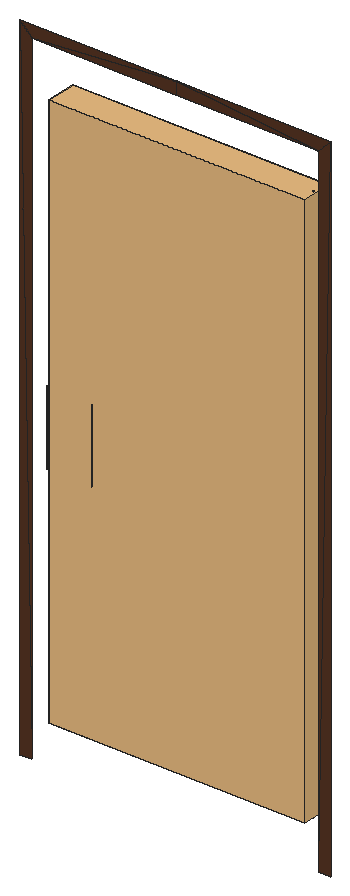
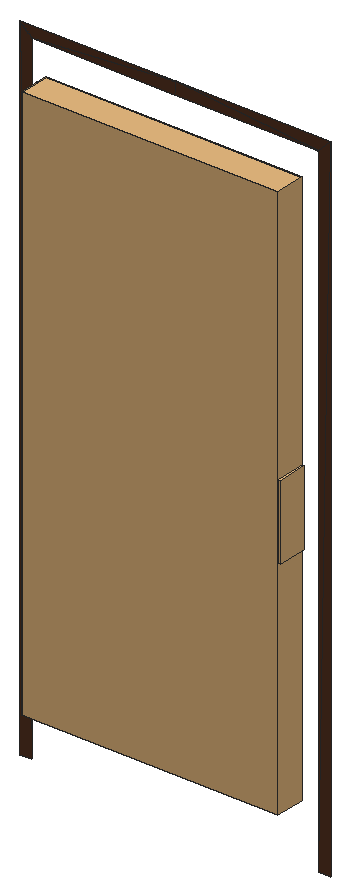
# SketchUp Ruby script. Lengths in inches.
U = 1.inch
M = Sketchup.active_model
def pt(a) = Geom::Point3d.new(a.map { |v| v * U })
def face(e, loops, mat)
  f = e.add_face(loops[0].map { |a| pt(a) })
  loops[1..].each { |l| e.add_face(l.map { |a| pt(a) }).erase! }
  f.material = f.back_material = mat if mat
  f
end
# faces: each face lists its corners as indices into pts; further lists are holes
def faces(e, pts, list, mat = nil) = list.each { |f| face(e, (f[0].is_a?(Array) ? f : [f]).map { |l| l.map { |i| pts[i] } }, mat) }
# xy, xz, yz: faces in a plane at the given z, y or x. An outline is a flat list of corners, or four numbers for a rectangle; further outlines are holes
def ring(l) = l.size == 4 ? [[l[0], l[1]], [l[2], l[1]], [l[2], l[3]], [l[0], l[3]]] : l.each_slice(2).to_a
def flat(e, list, mat, &to3) = list.each { |f| face(e, (f[0].is_a?(Array) ? f : [f]).map { |l| ring(l).map { |u, v| to3.(u, v) } }, mat) }
def xy(e, z, list, mat = nil) = flat(e, list, mat) { |x, y| [x, y, z] }
def xz(e, y, list, mat = nil) = flat(e, list, mat) { |x, z| [x, y, z] }
def yz(e, x, list, mat = nil) = flat(e, list, mat) { |y, z| [x, y, z] }
def lines(e, pts, list) = list.each { |a, b| e.add_line(pt(pts[a]), pt(pts[b])) }
# prism: a flat outline (further loops are holes) pulled along v
def prism(e, loops, v, mat = nil)
  f = face(e, loops, mat); d = Geom::Vector3d.new(v.map { |x| x * U })
  f.pushpull(f.normal.samedirection?(d) ? d.length : -d.length)
end
def box(e, o, s, mat = nil) = prism(e, [[o, [o[0] + s[0], o[1], o[2]], [o[0] + s[0], o[1] + s[1], o[2]], [o[0], o[1] + s[1], o[2]]]], [0, 0, s[2]], mat)
def at(x, y, z, deg = 0) = Geom::Transformation.translation(pt([x, y, z])) * Geom::Transformation.rotation(ORIGIN, Z_AXIS, deg.degrees)
def axes(o, x, y, z) = Geom::Transformation.new([*x, 0, *y, 0, *z, 0, *pt(o).to_a, 1])
def part(name) = M.definitions.add(name)
# library, detail: a bought-in or finely detailed component or shape, given as its bounding box
def library(name, o, s) = part(name).tap { |d| box(d.entities, o, s) }
def detail(e, o, s) = box(e.add_group.entities, o, s)
def put(e, d, t, mat = nil) = e.add_instance(d, t).tap { |i| i.material = mat if mat }
def group(e, t, mat = nil) = e.add_group.tap { |g| g.transformation = t; g.material = mat if mat }.entities
root = M.entities
M.materials.add("Material \#0").color = [86, 53, 35]
M.materials.add("Material \#1").color = [140, 140, 140]
c1 = part("3DGeom~8_Defintion")
xz(c1.entities,-471.94,[[458.125,-17.29,459.53,-16.11,457.73,-17.15],[458.125,-17.29,458.54,-17.29,459.53,-16.11],[458.54,-17.29,458.93,-17.15,459.53,-16.11],[457.73,-17.15,459.53,-16.11,457.42,-16.88],[458.93,-17.15,459.25,-16.88,459.53,-16.11],
  [457.42,-16.88,459.53,-16.11,457.21,-16.52],[459.25,-16.88,459.46,-16.52,459.53,-16.11],[457.21,-16.52,459.53,-16.11,457.14,-16.11],[457.14,-16.11,459.53,-16.11,457.21,-15.7],[459.53,-16.11,457.42,-15.34,457.21,-15.7],
  [459.53,-16.11,457.73,-15.07,457.42,-15.34],[459.53,-16.11,458.125,-14.93,457.73,-15.07],[459.53,-16.11,458.54,-14.93,458.125,-14.93],[459.53,-16.11,458.93,-15.07,458.54,-14.93],[459.53,-16.11,459.25,-15.34,458.93,-15.07],
  [459.53,-16.11,459.46,-15.7,459.25,-15.34]],"Material \#1")
xz(c1.entities,-416.39,[[458.125,-17.29,457.73,-17.15,459.53,-16.11],[458.125,-17.29,459.53,-16.11,458.54,-17.29],[458.54,-17.29,459.53,-16.11,458.93,-17.15],[457.73,-17.15,457.42,-16.88,459.53,-16.11],[458.93,-17.15,459.53,-16.11,459.25,-16.88],
  [457.42,-16.88,457.21,-16.52,459.53,-16.11],[459.25,-16.88,459.53,-16.11,459.46,-16.52],[457.21,-16.52,457.14,-16.11,459.53,-16.11],[457.14,-16.11,457.21,-15.7,459.53,-16.11],[459.53,-16.11,457.21,-15.7,457.42,-15.34],
  [459.53,-16.11,457.42,-15.34,457.73,-15.07],[459.53,-16.11,457.73,-15.07,458.125,-14.93],[459.53,-16.11,458.125,-14.93,458.54,-14.93],[459.53,-16.11,458.54,-14.93,458.93,-15.07],[459.53,-16.11,458.93,-15.07,459.25,-15.34],
  [459.53,-16.11,459.25,-15.34,459.46,-15.7]],"Material \#1")
xz(c1.entities,-27.5,[[458.125,-17.29,459.53,-16.11,457.73,-17.15],[458.125,-17.29,458.54,-17.29,459.53,-16.11],[458.54,-17.29,458.93,-17.15,459.53,-16.11],[457.73,-17.15,459.53,-16.11,457.42,-16.88],[458.93,-17.15,459.25,-16.88,459.53,-16.11],
  [457.42,-16.88,459.53,-16.11,457.21,-16.52],[459.25,-16.88,459.46,-16.52,459.53,-16.11],[457.21,-16.52,459.53,-16.11,457.14,-16.11],[457.14,-16.11,459.53,-16.11,457.21,-15.7],[459.53,-16.11,457.42,-15.34,457.21,-15.7],
  [459.53,-16.11,457.73,-15.07,457.42,-15.34],[459.53,-16.11,458.125,-14.93,457.73,-15.07],[459.53,-16.11,458.54,-14.93,458.125,-14.93],[459.53,-16.11,458.93,-15.07,458.54,-14.93],[459.53,-16.11,459.25,-15.34,458.93,-15.07],
  [459.53,-16.11,459.46,-15.7,459.25,-15.34]],"Material \#1")
xz(c1.entities,28.06,[[458.125,-17.29,457.73,-17.15,459.53,-16.11],[458.125,-17.29,459.53,-16.11,458.54,-17.29],[458.54,-17.29,459.53,-16.11,458.93,-17.15],[457.73,-17.15,457.42,-16.88,459.53,-16.11],[458.93,-17.15,459.53,-16.11,459.25,-16.88],
  [457.42,-16.88,457.21,-16.52,459.53,-16.11],[459.25,-16.88,459.53,-16.11,459.46,-16.52],[457.21,-16.52,457.14,-16.11,459.53,-16.11],[457.14,-16.11,457.21,-15.7,459.53,-16.11],[459.53,-16.11,457.21,-15.7,457.42,-15.34],
  [459.53,-16.11,457.42,-15.34,457.73,-15.07],[459.53,-16.11,457.73,-15.07,458.125,-14.93],[459.53,-16.11,458.125,-14.93,458.54,-14.93],[459.53,-16.11,458.54,-14.93,458.93,-15.07],[459.53,-16.11,458.93,-15.07,459.25,-15.34],
  [459.53,-16.11,459.25,-15.34,459.46,-15.7]],"Material \#1")
xz(c1.entities,472.5,[[458.125,-17.29,459.53,-16.11,457.73,-17.15],[458.125,-17.29,458.54,-17.29,459.53,-16.11],[458.54,-17.29,458.93,-17.15,459.53,-16.11],[457.73,-17.15,459.53,-16.11,457.42,-16.88],[458.93,-17.15,459.25,-16.88,459.53,-16.11],
  [457.42,-16.88,459.53,-16.11,457.21,-16.52],[459.25,-16.88,459.46,-16.52,459.53,-16.11],[457.21,-16.52,459.53,-16.11,457.14,-16.11],[457.14,-16.11,459.53,-16.11,457.21,-15.7],[459.53,-16.11,457.42,-15.34,457.21,-15.7],
  [459.53,-16.11,457.73,-15.07,457.42,-15.34],[459.53,-16.11,458.125,-14.93,457.73,-15.07],[459.53,-16.11,458.54,-14.93,458.125,-14.93],[459.53,-16.11,458.93,-15.07,458.54,-14.93],[459.53,-16.11,459.25,-15.34,458.93,-15.07],
  [459.53,-16.11,459.46,-15.7,459.25,-15.34]],"Material \#1")
xz(c1.entities,528.06,[[458.125,-17.29,457.73,-17.15,459.53,-16.11],[458.125,-17.29,459.53,-16.11,458.54,-17.29],[458.54,-17.29,459.53,-16.11,458.93,-17.15],[457.73,-17.15,457.42,-16.88,459.53,-16.11],[458.93,-17.15,459.53,-16.11,459.25,-16.88],
  [457.42,-16.88,457.21,-16.52,459.53,-16.11],[459.25,-16.88,459.53,-16.11,459.46,-16.52],[457.21,-16.52,457.14,-16.11,459.53,-16.11],[457.14,-16.11,457.21,-15.7,459.53,-16.11],[459.53,-16.11,457.21,-15.7,457.42,-15.34],
  [459.53,-16.11,457.42,-15.34,457.73,-15.07],[459.53,-16.11,457.73,-15.07,458.125,-14.93],[459.53,-16.11,458.125,-14.93,458.54,-14.93],[459.53,-16.11,458.54,-14.93,458.93,-15.07],[459.53,-16.11,458.93,-15.07,459.25,-15.34],
  [459.53,-16.11,459.25,-15.34,459.46,-15.7]],"Material \#1")
c2 = part("3DGeom~21_Defintion")
xy(c2.entities,73.08,[[-976.3,-241.71,23.7,-241.71,-976.3,-223.46],[23.7,-241.71,5.45,-223.46,-976.3,-223.46],[23.7,-241.71,23.7,0,5.45,-223.46],[5.45,-223.46,23.7,0,5.45,0],[23.7,0,23.7,241.71,5.45,223.46],
  [5.45,0,23.7,0,5.45,223.46],[-976.3,223.46,23.7,241.71,-976.3,241.71],[-976.3,223.46,5.45,223.46,23.7,241.71]],"Material \#0")
c3 = library("3DGeom~6_Defintion",[-5.59,-471.8,-48.03],[468.87,1000,73.72])
c4 = library("3DGeom~3_Defintion",[-83.33,-500,-350],[620.1,1000,533.33])
c5 = library("3DGeom~1_Defintion",[-60.87,347.29,-704.08],[121.74,121.75,1000])
c6 = library("3DGeom~13_Defintion",[-84.91,-744.98,-830.03],[169.82,169.83,1000])
xy(root,6.597,[[381.979,199.777,381.911,199.796,381.922,199.809],[381.979,199.777,381.922,199.809,381.983,199.793],[381.979,199.777,381.983,199.793,382.051,199.777],[382.051,199.777,381.983,199.793,382.047,199.793],[382.051,199.777,382.047,199.793,382.119,199.796],
  [382.047,199.793,382.108,199.809,382.119,199.796],[381.911,199.796,381.856,199.83,381.872,199.84],[381.911,199.796,381.872,199.84,381.922,199.809],[382.119,199.796,382.108,199.809,382.174,199.83],[382.108,199.809,382.158,199.84,382.174,199.83],
  [381.856,199.83,381.82,199.877,381.84,199.883],[381.856,199.83,381.84,199.883,381.872,199.84],[382.174,199.83,382.158,199.84,382.21,199.877],[382.158,199.84,382.19,199.883,382.21,199.877],[381.82,199.877,381.808,199.93,381.828,199.93],
  [381.82,199.877,381.828,199.93,381.84,199.883],[382.21,199.877,382.19,199.883,382.222,199.93],[382.19,199.883,382.201,199.93,382.222,199.93],[381.808,199.93,381.82,199.984,381.84,199.978],[381.808,199.93,381.84,199.978,381.828,199.93],
  [382.201,199.93,382.19,199.978,382.21,199.984],[382.201,199.93,382.21,199.984,382.222,199.93],[381.84,199.978,381.82,199.984,381.872,200.02],[382.19,199.978,382.158,200.02,382.174,200.03],[382.19,199.978,382.174,200.03,382.21,199.984],
  [381.82,199.984,381.856,200.03,381.872,200.02],[381.872,200.02,381.856,200.03,381.922,200.052],[382.158,200.02,382.108,200.052,382.119,200.065],[382.158,200.02,382.119,200.065,382.174,200.03],[381.856,200.03,381.911,200.065,381.922,200.052],
  [381.922,200.052,381.911,200.065,381.983,200.068],[382.108,200.052,382.047,200.068,382.051,200.084],[382.108,200.052,382.051,200.084,382.119,200.065],[381.911,200.065,381.979,200.084,381.983,200.068],[381.983,200.068,381.979,200.084,382.047,200.068],
  [382.047,200.068,381.979,200.084,382.051,200.084]],"Material \#1")
xy(root,6.614,[[381.979,199.777,381.983,199.793,381.911,199.796],[381.979,199.777,382.047,199.793,381.983,199.793],[381.979,199.777,382.051,199.777,382.047,199.793],[382.051,199.777,382.108,199.809,382.047,199.793],[382.051,199.777,382.119,199.796,382.108,199.809],
  [381.983,199.793,381.922,199.809,381.911,199.796],[381.911,199.796,381.922,199.809,381.856,199.83],[382.119,199.796,382.158,199.84,382.108,199.809],[382.119,199.796,382.174,199.83,382.158,199.84],[381.922,199.809,381.872,199.84,381.856,199.83],
  [381.856,199.83,381.872,199.84,381.82,199.877],[382.174,199.83,382.19,199.883,382.158,199.84],[382.174,199.83,382.21,199.877,382.19,199.883],[381.872,199.84,381.84,199.883,381.82,199.877],[381.82,199.877,381.84,199.883,381.808,199.93],
  [382.21,199.877,382.201,199.93,382.19,199.883],[382.21,199.877,382.222,199.93,382.201,199.93],[381.84,199.883,381.828,199.93,381.808,199.93],[381.808,199.93,381.828,199.93,381.82,199.984],[381.828,199.93,381.84,199.978,381.82,199.984],
  [382.201,199.93,382.222,199.93,382.19,199.978],[382.222,199.93,382.21,199.984,382.19,199.978],[381.84,199.978,381.856,200.03,381.82,199.984],[381.84,199.978,381.872,200.02,381.856,200.03],[382.19,199.978,382.21,199.984,382.158,200.02],
  [382.21,199.984,382.174,200.03,382.158,200.02],[381.872,200.02,381.911,200.065,381.856,200.03],[381.872,200.02,381.922,200.052,381.911,200.065],[382.158,200.02,382.174,200.03,382.108,200.052],[382.174,200.03,382.119,200.065,382.108,200.052],
  [381.922,200.052,381.979,200.084,381.911,200.065],[381.922,200.052,381.983,200.068,381.979,200.084],[382.108,200.052,382.119,200.065,382.047,200.068],[382.119,200.065,382.051,200.084,382.047,200.068],[381.983,200.068,382.051,200.084,381.979,200.084],
  [381.983,200.068,382.047,200.068,382.051,200.084]],"Material \#1")
xy(root,10.426,[[381.979,199.777,381.911,199.796,381.983,199.793],[381.979,199.777,381.983,199.793,382.047,199.793],[381.979,199.777,382.047,199.793,382.051,199.777],[382.051,199.777,382.047,199.793,382.108,199.809],[382.051,199.777,382.108,199.809,382.119,199.796],
  [381.983,199.793,381.911,199.796,381.922,199.809],[381.911,199.796,381.856,199.83,381.922,199.809],[382.119,199.796,382.108,199.809,382.158,199.84],[382.119,199.796,382.158,199.84,382.174,199.83],[381.922,199.809,381.856,199.83,381.872,199.84],
  [381.856,199.83,381.82,199.877,381.872,199.84],[382.174,199.83,382.158,199.84,382.19,199.883],[382.174,199.83,382.19,199.883,382.21,199.877],[381.872,199.84,381.82,199.877,381.84,199.883],[381.82,199.877,381.808,199.93,381.84,199.883],
  [382.21,199.877,382.19,199.883,382.201,199.93],[382.21,199.877,382.201,199.93,382.222,199.93],[381.84,199.883,381.808,199.93,381.828,199.93],[381.808,199.93,381.82,199.984,381.828,199.93],[381.828,199.93,381.82,199.984,381.84,199.978],
  [382.201,199.93,382.19,199.978,382.222,199.93],[382.222,199.93,382.19,199.978,382.21,199.984],[381.84,199.978,381.82,199.984,381.856,200.03],[381.84,199.978,381.856,200.03,381.872,200.02],[382.19,199.978,382.158,200.02,382.21,199.984],
  [382.21,199.984,382.158,200.02,382.174,200.03],[381.872,200.02,381.856,200.03,381.911,200.065],[381.872,200.02,381.911,200.065,381.922,200.052],[382.158,200.02,382.108,200.052,382.174,200.03],[382.174,200.03,382.108,200.052,382.119,200.065],
  [381.922,200.052,381.911,200.065,381.979,200.084],[381.922,200.052,381.979,200.084,381.983,200.068],[382.108,200.052,382.047,200.068,382.119,200.065],[382.119,200.065,382.047,200.068,382.051,200.084],[381.983,200.068,381.979,200.084,382.051,200.084],
  [381.983,200.068,382.051,200.084,382.047,200.068]],"Material \#1")
xy(root,10.443,[[381.979,199.777,381.922,199.809,381.911,199.796],[381.979,199.777,381.983,199.793,381.922,199.809],[381.979,199.777,382.051,199.777,381.983,199.793],[382.051,199.777,382.047,199.793,381.983,199.793],[382.051,199.777,382.119,199.796,382.047,199.793],
  [382.047,199.793,382.119,199.796,382.108,199.809],[381.911,199.796,381.872,199.84,381.856,199.83],[381.911,199.796,381.922,199.809,381.872,199.84],[382.119,199.796,382.174,199.83,382.108,199.809],[382.108,199.809,382.174,199.83,382.158,199.84],
  [381.856,199.83,381.84,199.883,381.82,199.877],[381.856,199.83,381.872,199.84,381.84,199.883],[382.174,199.83,382.21,199.877,382.158,199.84],[382.158,199.84,382.21,199.877,382.19,199.883],[381.82,199.877,381.828,199.93,381.808,199.93],
  [381.82,199.877,381.84,199.883,381.828,199.93],[382.21,199.877,382.222,199.93,382.19,199.883],[382.19,199.883,382.222,199.93,382.201,199.93],[381.808,199.93,381.828,199.93,381.84,199.978],[381.808,199.93,381.84,199.978,381.82,199.984],
  [382.201,199.93,382.21,199.984,382.19,199.978],[382.201,199.93,382.222,199.93,382.21,199.984],[381.84,199.978,381.872,200.02,381.82,199.984],[382.19,199.978,382.174,200.03,382.158,200.02],[382.19,199.978,382.21,199.984,382.174,200.03],
  [381.82,199.984,381.872,200.02,381.856,200.03],[381.872,200.02,381.922,200.052,381.856,200.03],[382.158,200.02,382.119,200.065,382.108,200.052],[382.158,200.02,382.174,200.03,382.119,200.065],[381.856,200.03,381.922,200.052,381.911,200.065],
  [381.922,200.052,381.983,200.068,381.911,200.065],[382.108,200.052,382.051,200.084,382.047,200.068],[382.108,200.052,382.119,200.065,382.051,200.084],[381.911,200.065,381.983,200.068,381.979,200.084],[381.983,200.068,382.047,200.068,381.979,200.084],
  [382.047,200.068,382.051,200.084,381.979,200.084]],"Material \#1")
xy(root,40.624,[[347.812,200.864,347.812,201.153,347.848,200.864],[347.848,200.864,347.812,201.153,347.848,201.153]],"Material \#1")
xy(root,40.964,[[347.794,200.864,347.854,200.864,347.854,201.153]],"Material \#1")
xz(root,200.833,[[347.824,40.059,347.893,40.076,347.86,40.064],[347.754,40.076,347.977,40.184,347.893,40.076],[347.893,40.076,347.947,40.12,347.922,40.095],[347.893,40.076,347.977,40.184,347.947,40.12],[347.947,40.12,347.977,40.184,347.965,40.15],
  [347.977,40.184,347.66,40.554,347.981,40.221],[347.981,40.221,347.767,40.546,347.824,40.539],[347.981,40.221,347.824,40.539,347.881,40.546],[347.981,40.221,347.881,40.546,347.981,40.53],[347.981,40.53,347.881,40.546,347.983,40.543],
  [347.981,40.53,347.983,40.543,347.982,40.537],[347.983,40.543,347.881,40.546,347.988,40.555],[347.983,40.543,347.988,40.555,347.985,40.549],[347.881,40.546,347.933,40.565,347.988,40.555],[347.988,40.555,347.933,40.565,347.979,40.595],
  [347.988,40.555,347.979,40.595,348.018,40.635],[347.988,40.555,348.018,40.635,348.103,40.756],[347.988,40.555,348.103,40.756,347.991,40.56],[347.991,40.56,348.103,40.756,347.995,40.565],[347.995,40.565,348.048,40.623,348,40.57],
  [347.995,40.565,348.103,40.756,348.048,40.623],[348,40.57,348.048,40.623,348.026,40.595],[348.048,40.623,348.084,40.685,348.068,40.653],[348.048,40.623,348.103,40.756,348.084,40.685],[348.018,40.635,348.047,40.682,348.103,40.756],
  [348.047,40.682,348.066,40.736,348.103,40.756],[348.084,40.685,348.103,40.756,348.096,40.72],[348.066,40.736,348.072,40.794,348.103,40.756],[348.103,40.756,348.044,40.975,348.098,40.861],[348.103,40.756,348.066,40.853,348.044,40.975],
  [348.103,40.756,348.072,40.794,348.066,40.853],[348.103,40.756,348.098,40.861,348.105,40.794],[348.066,40.853,348.047,40.906,348.044,40.975],[348.098,40.861,348.044,40.975,348.077,40.921],[348.047,40.906,348.018,40.954,348.044,40.975],
  [348.018,40.954,347.979,40.993,348.044,40.975],[348.044,40.975,347.824,41.083,347.948,41.054],[348.044,40.975,347.933,41.023,347.824,41.083],[348.044,40.975,347.979,40.993,347.933,41.023],[348.044,40.975,347.948,41.054,348,41.02],
  [347.933,41.023,347.881,41.043,347.824,41.083],[347.881,41.043,347.824,41.049,347.824,41.083],[347.948,41.054,347.824,41.083,347.888,41.076]],"Material \#1")
xz(root,201.113,[[348.378,37.766,348.439,37.876,348.368,37.774],[348.378,37.766,348.45,37.87,348.439,37.876],[348.032,37.823,348.049,37.861,348.038,37.866],[348.049,37.861,348.048,37.905,348.038,37.866],[348.049,37.861,348.061,37.903,348.048,37.905],
  [348.45,37.87,348.491,37.99,348.439,37.876],[348.45,37.87,348.503,37.986,348.491,37.99],[348.065,37.947,348.061,37.991,348.048,37.989],[348.503,37.986,348.525,38.113,348.491,37.99],[348.503,37.986,348.537,38.111,348.525,38.113],
  [348.048,37.989,348.061,37.991,348.038,38.029],[348.061,37.991,348.049,38.033,348.038,38.029],[348.537,38.111,348.537,38.25,348.525,38.113],[348.537,38.111,348.549,38.249,348.537,38.25],[348.549,38.249,348.537,44.909,348.537,38.25],
  [348.549,38.249,348.537,46.738,348.537,44.909],[348.549,38.249,348.549,46.739,348.537,46.738]],"Material \#1")
yz(root,347.848,[[200.864,40.718,201.153,40.718,200.864,40.748],[201.153,40.718,201.153,40.748,200.864,40.748]],"Material \#1")
yz(root,347.854,[[200.864,40.837,201.153,40.837,200.864,40.892]],"Material \#1")
yz(root,347.857,[[200.864,40.772,201.153,40.772,200.864,40.796],[201.153,40.772,201.153,40.796,200.864,40.796]],"Material \#1")
p = [[347.741,201.113,37.876],[347.722,201.106,37.849],[347.722,201.081,37.849],[347.741,201.088,37.876],[347.743,201.106,37.83],[347.743,201.081,37.83],
  [347.769,201.106,37.816],[347.769,201.081,37.816],[347.787,201.113,37.843],[347.787,201.088,37.843],[347.803,201.116,37.867],[347.803,201.091,37.867],
  [347.757,201.116,37.899],[347.757,201.091,37.9],[347.845,201.116,38.028],[347.845,201.091,38.028],[347.891,201.116,37.995],[347.891,201.091,37.995],
  [347.861,201.113,38.052],[347.861,201.088,38.052],[347.907,201.113,38.019],[347.907,201.088,38.019],[347.925,201.106,38.045],[347.925,201.081,38.045],
  [347.904,201.106,38.065],[347.904,201.081,38.065],[347.879,201.106,38.078],[347.879,201.081,38.078],[347.839,201.153,40.654],[347.842,200.864,40.658],
  [347.836,200.864,40.65],[347.836,200.864,40.65],[347.848,200.864,40.624],[347.848,201.153,40.624],[347.848,201.153,40.624],[347.839,201.153,40.654],
  [347.836,200.864,40.65],[347.848,200.864,40.718],[347.836,200.864,40.686],[347.839,201.153,40.682],[347.839,201.153,40.682],[347.836,200.864,40.686],
  [347.842,200.864,40.678],[347.848,201.153,40.748],[347.857,201.153,40.772],[347.857,200.864,40.772],[347.848,200.864,40.748],[347.839,201.153,40.654],
  [347.839,201.153,40.682],[347.842,200.864,40.678],[347.842,200.864,40.658],[347.839,201.153,40.682],[347.848,201.153,40.718],[347.848,200.864,40.718],
  [347.848,200.864,40.82],[347.857,200.864,40.796],[347.857,201.153,40.796],[347.854,200.864,40.837],[347.848,200.864,40.82],[347.848,201.153,40.82],
  [347.857,201.153,40.796],[347.848,201.153,40.82],[347.848,200.864,40.82],[347.848,201.153,40.82],[347.854,201.153,40.837],[347.854,200.864,40.837],
  [347.854,201.153,40.837],[347.851,201.153,40.902],[347.854,200.864,40.892],[347.854,200.864,40.964],[347.854,200.864,40.909],[347.851,201.153,40.902],
  [347.851,201.153,40.902],[347.854,201.153,40.964],[347.854,200.864,40.964]]
faces(root,p,[[0,1,2],[2,3,0],[1,4,5],[5,2,1],[4,6,7],[7,5,4],[6,8,9],[9,7,6],
  [8,10,11],[11,9,8],[12,0,3],[3,13,12],[14,12,13],[13,15,14],[10,16,17],[17,11,10],
  [18,14,15],[15,19,18],[16,20,21],[21,17,16],[20,22,23],[23,21,20],[22,24,25],[25,23,22],
  [24,26,27],[27,25,24],[26,18,19],[19,27,26],[28,29,30],[31,32,33],[34,35,36],[37,38,39],
  [40,41,42],[43,44,45],[45,46,43],[47,48,49],[49,50,47],[51,52,53],[54,55,56],[57,58,59],
  [60,61,62],[63,64,65],[66,67,68],[69,70,71],[72,73,74]],"Material \#1")
put(root,c1,axes([347.82,200.83,42.49],[0.0746,0,0],[0,0,0.07649],[0,0.05601,0]),"Material \#1")
put(root,c2,axes([363.16,204.75,87.54],[0,0,0.08966],[0.08745,0,0],[0,-0.06565,0]),"Material \#0")
put(root,c3,axes([347.82,200.83,42.49],[0.07421,0,0],[0,0,0.07609],[0,0.05571,0]),"Material \#1")
put(root,c4,axes([347.82,200.83,42.49],[0.00995,0,0],[0,0,0.0102],[0,0.00747,0]),"Material \#1")
put(root,c5,axes([347.82,200.83,42.49],[0.00406,0,0],[0,0,0.00416],[0,0.00305,0]),"Material \#1")
put(root,c6,axes([347.82,200.83,42.49],[0.00251,0,0],[0,0,0.00258],[0,0.00189,0]),"Material \#1")
